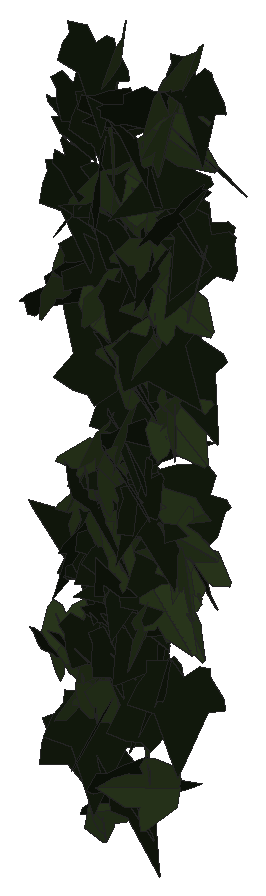
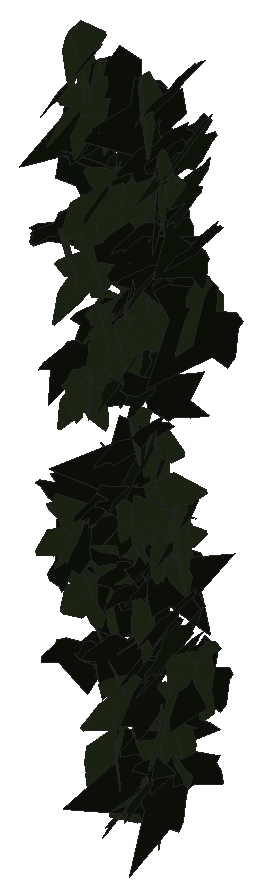
# SketchUp Ruby script. Lengths in inches.
U = 1.inch
M = Sketchup.active_model
def pt(a) = Geom::Point3d.new(a.map { |v| v * U })
def face(e, loops, mat)
  f = e.add_face(loops[0].map { |a| pt(a) })
  loops[1..].each { |l| e.add_face(l.map { |a| pt(a) }).erase! }
  f.material = f.back_material = mat if mat
  f
end
# faces: each face lists its corners as indices into pts; further lists are holes
def faces(e, pts, list, mat = nil) = list.each { |f| face(e, (f[0].is_a?(Array) ? f : [f]).map { |l| l.map { |i| pts[i] } }, mat) }
# xy, xz, yz: faces in a plane at the given z, y or x. An outline is a flat list of corners, or four numbers for a rectangle; further outlines are holes
def ring(l) = l.size == 4 ? [[l[0], l[1]], [l[2], l[1]], [l[2], l[3]], [l[0], l[3]]] : l.each_slice(2).to_a
def flat(e, list, mat, &to3) = list.each { |f| face(e, (f[0].is_a?(Array) ? f : [f]).map { |l| ring(l).map { |u, v| to3.(u, v) } }, mat) }
def xy(e, z, list, mat = nil) = flat(e, list, mat) { |x, y| [x, y, z] }
def xz(e, y, list, mat = nil) = flat(e, list, mat) { |x, z| [x, y, z] }
def yz(e, x, list, mat = nil) = flat(e, list, mat) { |y, z| [x, y, z] }
def lines(e, pts, list) = list.each { |a, b| e.add_line(pt(pts[a]), pt(pts[b])) }
# prism: a flat outline (further loops are holes) pulled along v
def prism(e, loops, v, mat = nil)
  f = face(e, loops, mat); d = Geom::Vector3d.new(v.map { |x| x * U })
  f.pushpull(f.normal.samedirection?(d) ? d.length : -d.length)
end
def box(e, o, s, mat = nil) = prism(e, [[o, [o[0] + s[0], o[1], o[2]], [o[0] + s[0], o[1] + s[1], o[2]], [o[0], o[1] + s[1], o[2]]]], [0, 0, s[2]], mat)
def at(x, y, z, deg = 0) = Geom::Transformation.translation(pt([x, y, z])) * Geom::Transformation.rotation(ORIGIN, Z_AXIS, deg.degrees)
def axes(o, x, y, z) = Geom::Transformation.new([*x, 0, *y, 0, *z, 0, *pt(o).to_a, 1])
def part(name) = M.definitions.add(name)
# library, detail: a bought-in or finely detailed component or shape, given as its bounding box
def library(name, o, s) = part(name).tap { |d| box(d.entities, o, s) }
def detail(e, o, s) = box(e.add_group.entities, o, s)
def put(e, d, t, mat = nil) = e.add_instance(d, t).tap { |i| i.material = mat if mat }
def group(e, t, mat = nil) = e.add_group.tap { |g| g.transformation = t; g.material = mat if mat }.entities
root = M.entities
M.materials.add("efeu1").color = [18, 25, 13]
M.materials.add("efeu2").color = [43, 57, 29]
c1 = part("ivyleaf_10")
p = [[0,0.5,-0.03],[-0.0625,2.02,-0.43],[-0.19,2.01,-0.46],[-0.54,1.05,-0.29],[-0.52,0.625,-0.18],[-0.83,0.76,-0.28],
  [-1.16,0.64,-0.33],[-1.15,0.33,-0.24],[-0.77,-0.39,0.02],[-0.3,-0.51,0.16],[0.04,-0.48,0.23],[-0.02,2.01,-0.4375],
  [-0.06,2.01,-0.43],[0.04,-0.49,0.23],[0.67,-0.49,0.14],[1.38,0.36,-0.2],[1.375,0.51,-0.24],[0.81,0.65,-0.19],
  [0.62,0.59,-0.15],[0.6,1.09,-0.28],[0.5,1.23,-0.31]]
faces(c1.entities,p,[[0,1,2,3,4,5,6,7,8,9,10],[11,12,0,13,14,15,16,17,18,19,20]],"efeu2")
c2 = part("ivyleaf_9")
p = [[1.54,2.16,1.25],[1.36,2.04,1.19],[-0.21,0.99,0.68],[-0.71,1.11,0.82],[-0.85,0.86,0.67],[-0.8,0.17,0.21],
  [-0.9,-0.01,0.1],[-0.67,-0.16,-0.02],[-0.08,-0.08,-0.05],[-0.03,-0.6,-0.4],[0.65,-0.88,-0.66],[0.83,-0.6,-0.49],
  [1.29,-0.42,-0.43],[1.8125,-0.07,-0.26],[1.21,0.44,0.15]]
faces(c2.entities,p,[[0,1,2,3,4,5,6,7,8,9,10,11,12,13,14]],"efeu1")
put(root,c1,axes([531.04,134.63,192.66],[0.26361,-0.71139,-0.19754],[-0.06426,0.18685,-0.75865],[0.73551,0.27129,0.00452]))
put(root,c2,axes([530.74,133.59,188.14],[0.75303,0.05984,-0.12105],[-0.12035,-0.01367,-0.75539],[-0.06125,0.76257,-0.00404]))
put(root,c2,axes([530.68,134.68,201.09],[0.16312,-0.82332,-0.03787],[-0.0011,0.03838,-0.8393],[0.82419,0.16299,0.00638]))
put(root,c2,axes([530.67,135.42,189.45],[0.04193,-0.62521,0.47513],[0.1896,-0.45367,-0.6137],[0.76203,0.14728,0.12655]))
put(root,c2,axes([530.9,133.39,198.6],[0.47981,0.7112,0.3862],[0.22324,0.31524,-0.85788],[-0.77789,0.52914,-0.00799]))
put(root,c1,axes([531.09,133.39,198.99],[-0.052,-0.49853,-0.72888],[0.08284,0.72417,-0.50121],[0.87917,-0.09772,0.00412]))
put(root,c1,axes([530.52,134.08,187.91],[0.10779,-0.17311,0.79881],[0.78917,-0.1877,-0.14717],[0.21277,0.78389,0.14117]))
put(root,c2,axes([531.32,133.77,200.6875],[0.21484,0.45839,0.65824],[0.01162,0.67959,-0.47705],[-0.80204,0.13264,0.16941]))
put(root,c1,axes([531.1,133.67,188.23],[0.32155,0.28852,-0.63424],[0.19396,0.63384,0.38668],[0.66924,-0.32233,0.19267]))
put(root,c1,axes([531.3,134.66,192.12],[-0.11723,-0.743,0.24242],[0.02821,-0.249,-0.74951],[0.78104,-0.10253,0.06345]))
put(root,c2,axes([531.81,134.42,190.58],[-0.00979,0.0925,0.81453],[-0.81733,0.06158,-0.01681],[-0.06308,-0.81226,0.09148]))
put(root,c2,axes([530.92,134.39,203.95],[0.45755,-0.69505,-0.09896],[-0.04108,0.09141,-0.83198],[0.70085,0.45912,0.01584]))
put(root,c2,axes([531.51,134.39,191.29],[-0.22531,0.51676,-0.53556],[0.20531,-0.49469,-0.5637],[-0.71534,-0.30475,0.00689]))
put(root,c1,axes([531.23,135.18,186.88],[-0.20489,0.5131,-0.49031],[0.08671,-0.48841,-0.54735],[-0.70438,-0.20937,0.07524]))
put(root,c2,axes([531.09,134.95,190.23],[0.19405,-0.73731,-0.05239],[-0.01151,0.05115,-0.76241],[0.73908,0.19438,0.00188]))
put(root,c1,axes([531.49,134.24,186.61],[0.08974,-0.89177,0.10539],[0.0243,-0.10347,-0.89616],[0.89764,0.09195,0.01373]))
put(root,c1,axes([531.67,134.61,193.43],[-0.44438,-0.65768,0.26278],[-0.05845,-0.27511,-0.78738],[0.70582,-0.43686,0.10025]))
put(root,c2,axes([532.08,134.54,196.17],[-0.78986,-0.33319,-0.19865],[-0.16849,-0.11122,0.8565],[-0.34941,0.80683,0.03603]))
put(root,c1,axes([531.67,134.48,191.43],[-0.44472,0.70787,-0.06223],[-0.0388,0.04911,0.83595],[0.70954,0.44635,0.00671]))
put(root,c2,axes([531.26,134.28,185.53],[-0.20793,-0.59761,-0.51311],[0.2079,0.47022,-0.63191],[0.75973,-0.29224,0.03249]))
put(root,c2,axes([531.3,133.41,203.66],[0.75435,-0.07109,-0.35592],[-0.28107,0.40497,-0.6766],[0.22964,0.7292,0.34106]))
put(root,c2,axes([531.41,134.5,184.7],[0.76234,-0.0328,-0.37748],[-0.37478,0.05955,-0.76205],[0.05577,0.84859,0.03888]))
put(root,c2,axes([531.26,133.6875,202.3],[0.65749,-0.42141,-0.2776],[-0.15246,0.26875,-0.76907],[0.48104,0.66116,0.13568]))
put(root,c1,axes([531.87,133.5625,187.26],[-0.12224,0.26561,0.72242],[-0.37787,0.61655,-0.29062],[-0.67056,-0.39585,0.03207]))
put(root,c2,axes([531.15,134.58,192.52],[0.54429,-0.78141,0.18703],[0.09921,-0.15881,-0.95225],[0.79733,0.55318,-0.00919]))
put(root,c2,axes([531.48,134.15,188.61],[0.36869,-0.62159,-0.33271],[-0.06126,0.34579,-0.71392],[0.70237,0.35645,0.11238]))
put(root,c2,axes([532.01,133.43,185.53],[0.05249,0.44209,0.63564],[0.02991,0.63547,-0.44444],[-0.77368,0.05456,0.02594]))
put(root,c2,axes([531.58,134.4,205.38],[0.10788,-0.82442,0.12259],[0.03031,-0.11965,-0.83133],[0.83294,0.11113,0.01438]))
put(root,c2,axes([531.61,134.8,191.22],[0.18444,-0.76454,-0.04074],[-0.00089,0.04169,-0.78642],[0.76562,0.18423,0.0089]))
put(root,c1,axes([532.01,134.82,205.35],[0.31164,-0.76022,-0.18841],[-0.00721,0.19998,-0.81884],[0.78318,0.30434,0.06744]))
put(root,c1,axes([532.11,134.15,202.97],[0.62794,-0.42437,-0.34252],[-0.13933,0.38019,-0.72647],[0.52725,0.60587,0.21595]))
put(root,c1,axes([532.32,133.64,183.4],[-0.12445,0.42105,-0.59435],[-0.26445,0.5357,0.43488],[0.67868,0.28594,0.06046]))
put(root,c2,axes([532.43,133.46,202.3],[0.03549,0.0188,-0.84588],[-0.74612,0.39992,-0.02242],[0.39897,0.74622,0.03332]))
put(root,c2,axes([531.92,134.18,186.125],[-0.28677,-0.81797,-0.1913],[0.07166,0.17758,-0.86674],[0.83698,-0.29546,0.00866]))
put(root,c1,axes([532.15,134.09,194.47],[0.06954,-0.75524,-0.18981],[0.03256,0.19322,-0.75687],[0.77804,0.05942,0.04864]))
put(root,c2,axes([531.78,134.27,199.75],[-0.04392,-0.58968,-0.56458],[0.19988,0.54042,-0.58],[0.79153,-0.16919,0.11513]))
put(root,c2,axes([532.61,135.1875,200.28],[-0.2321,-0.07874,0.763],[-0.71754,-0.25948,-0.24505],[0.27112,-0.75413,0.00465]))
put(root,c2,axes([531.8,134.7,201.48],[0.13318,-0.79396,-0.27331],[0.02514,0.28038,-0.80223],[0.83931,0.11759,0.0674]))
put(root,c2,axes([531.91,134.52,203.66],[0.02856,-0.81659,-0.19197],[-0.02894,0.19101,-0.81681],[0.83835,0.03441,-0.02166]))
put(root,c1,axes([531.91,134.41,191.91],[-0.50659,0.31057,-0.50559],[0.35044,-0.37986,-0.58447],[-0.47882,-0.6066,0.10715]))
put(root,c1,axes([532,134.92,189.29],[0.06572,-0.35407,-0.79019],[0.12113,-0.78091,0.35999],[-0.85738,-0.13747,-0.00971]))
put(root,c1,axes([532.29,134.93,193.07],[0.02918,-0.79936,0.0857],[0.00696,-0.0855,-0.79989],[0.80391,0.02976,0.00381]))
put(root,c2,axes([531.875,134.6875,199.97],[0.52852,-0.60117,-0.18155],[-0.0864,0.16542,-0.7993],[0.62202,0.53379,0.04324]))
put(root,c1,axes([532.4,134.27,186.95],[-0.49121,-0.65682,0.02553],[-0.01525,-0.02047,-0.82018],[0.65714,-0.49144,0.00004]))
put(root,c2,axes([532.77,135.22,193.18],[-0.61578,-0.06983,0.43979],[-0.42106,-0.15294,-0.61384],[0.14492,-0.74109,0.08524]))
put(root,c1,axes([532.6,134.06,191.27],[0.53556,-0.23189,-0.50994],[-0.47349,0.18962,-0.58351],[0.29936,0.71478,-0.01063]))
put(root,c1,axes([532.1875,134.09,198.66],[-0.26712,-0.54805,-0.55714],[0.29128,0.47655,-0.60842],[0.72521,-0.39327,0.03916]))
put(root,c1,axes([532.48,134.04,202],[-0.30002,-0.84663,0.00578],[-0.00184,-0.00548,-0.89821],[0.84665,-0.30002,0.0001]))
put(root,c2,axes([532.01,134.56,184.82],[0.51688,-0.65093,-0.05961],[-0.03879,0.04531,-0.83118],[0.6525,0.51833,-0.0022]))
put(root,c2,axes([531.99,135.25,194.22],[0.27883,-0.66473,0.43253],[0.147,-0.40722,-0.7206],[0.77932,0.31464,-0.01883]))
put(root,c1,axes([532.08,134.1,197.89],[0.68651,0.11248,-0.49154],[0.48576,0.07522,0.69565],[0.13527,-0.84098,-0.00352]))
put(root,c2,axes([531.96,134.53,187.5625],[0.82858,-0.34182,0.18948],[0.16868,-0.08788,-0.89616],[0.35254,0.84541,-0.01654]))
put(root,c2,axes([532.42,134.72,190.6],[-0.16663,-0.761,0.11539],[-0.00295,-0.11743,-0.77872],[0.76969,-0.1652,0.02199]))
put(root,c2,axes([532.19,134.58,200.71],[0.21458,-0.77793,0.15754],[0.07278,-0.14323,-0.80637],[0.79038,0.22439,0.03148]))
put(root,c2,axes([532.35,134.95,195.01],[-0.03554,-0.79116,-0.10623],[0.01827,0.1055,-0.79184],[0.79805,-0.03765,0.0134]))
put(root,c2,axes([532.39,134.5,190.86],[-0.31651,-0.60485,-0.43687],[0.18613,0.39554,-0.68248],[0.72253,-0.36686,-0.01556]))
put(root,c2,axes([532.23,134.58,193.125],[0.43206,-0.62245,-0.24071],[-0.07004,0.24287,-0.75377],[0.66368,0.43085,0.07715]))
put(root,c1,axes([532.7,133.45,193.68],[-0.18292,0.53797,0.53709],[-0.22845,0.48799,-0.56659],[-0.72505,-0.28948,0.04302]))
put(root,c2,axes([532.34,134.22,188.34],[0.30193,-0.69926,-0.17699],[-0.08116,0.15771,-0.76157],[0.71672,0.31243,-0.01169]))
put(root,c2,axes([532.14,134.38,196.73],[0.59211,-0.54134,0.14898],[0.11064,-0.09978,-0.80227],[0.55046,0.60235,0.001]))
put(root,c2,axes([532.73,134.27,189.03],[0.62248,-0.05553,0.53195],[-0.52657,0.07936,0.62447],[-0.09369,-0.81496,0.02456]))
put(root,c2,axes([532.11,133.76,203.85],[0.55006,0.15062,0.6169],[0.57939,0.21502,-0.56911],[-0.25992,0.79806,0.0369]))
put(root,c1,axes([532.38,133.58,183.77],[-0.0735,-0.08981,-0.73061],[0.46458,0.56387,-0.11605],[0.57098,-0.47036,0.00038]))
put(root,c1,axes([532.86,134.39,201.42],[-0.76252,-0.26645,0.11069],[-0.11263,-0.01306,-0.80736],[0.26564,-0.7704,-0.0246]))
put(root,c1,axes([532.68,134.33,194.93],[0.37753,-0.68155,0.1673],[0.08185,-0.14592,-0.77912],[0.69699,0.3863,0.00087]))
put(root,c2,axes([532.58,134.81,188.84],[-0.11024,-0.68489,-0.45434],[0.08855,0.44584,-0.69357],[0.8171,-0.14072,0.01386]))
put(root,c2,axes([532.36,134.39,193.38],[0.28643,-0.50862,0.53213],[0.30968,-0.43475,-0.58223],[0.6678,0.41976,0.04176]))
put(root,c1,axes([532.59,134.5,187.11],[-0.34134,-0.27715,-0.64569],[0.5212,0.38158,-0.43931],[0.47126,-0.62276,0.01818]))
put(root,c2,axes([532.4,134.35,193.83],[0.43906,0.11727,0.70979],[0.6632,0.25625,-0.45257],[-0.27878,0.7943,0.04121]))
put(root,c1,axes([533.08,134.81,197.66],[-0.34941,-0.67022,0.29406],[-0.00808,-0.3223,-0.74419],[0.73185,-0.32355,0.13218]))
put(root,c2,axes([532.56,133.5,184.28],[0.52369,0.38051,0.68488],[0.53127,0.43301,-0.6468],[-0.57585,0.74553,0.02611]))
put(root,c2,axes([532.51,134.52,203.12],[0.16561,-0.57207,0.58879],[0.30832,-0.51334,-0.58548],[0.76084,0.33254,0.1091]))
put(root,c2,axes([532.82,133.9375,199.03],[0.37706,-0.51834,-0.57077],[-0.29889,0.48742,-0.64009],[0.71072,0.47998,0.03362]))
put(root,c2,axes([532.625,134.56,184.05],[0.35268,-0.73903,0.03827],[0.01741,-0.0341,-0.81887],[0.73981,0.3531,0.00102]))
put(root,c2,axes([533.66,134.49,190.55],[-0.71863,0.06407,0.43761],[-0.4387,0.00266,-0.72081],[-0.05611,-0.84138,0.03104]))
put(root,c2,axes([532.9,134.83,188.45],[-0.29988,-0.57735,0.46408],[0.09329,-0.52612,-0.59425],[0.73485,-0.16882,0.26482]))
put(root,c2,axes([532.5625,134.54,192.59],[0.7129,-0.30211,0.154],[0.13724,-0.07078,-0.77419],[0.31008,0.7259,-0.01139]))
put(root,c1,axes([533.13,134.39,198.24],[-0.01812,-0.74129,0.37323],[0.07153,-0.37332,-0.738],[0.82685,0.01605,0.07202]))
put(root,c1,axes([533.38,133.91,197.1],[-0.73795,-0.28634,0.22004],[-0.18699,-0.12528,-0.79014],[0.30893,-0.7598,0.04736]))
put(root,c1,axes([532.74,134.98,185.38],[0.0457,-0.17408,0.78669],[0.64452,-0.46496,-0.14033],[0.48351,0.63623,0.1127]))
put(root,c2,axes([532.8,134.74,196.67],[0.3601,-0.7032,0.15678],[0.04934,-0.15079,-0.78967],[0.71878,0.36265,-0.02434]))
put(root,c1,axes([533.77,134.38,184.51],[-0.06632,-0.04578,-0.84309],[-0.68978,-0.48478,0.08058],[-0.48693,0.69296,0.00067]))
put(root,c1,axes([533.21,134.59,190.77],[-0.78939,-0.00174,0.28742],[0.28741,-0.01148,0.78931],[0.00229,0.84001,0.01138]))
put(root,c2,axes([532.97,134.47,199.91],[-0.18167,-0.01208,-0.80373],[0.80324,-0.03401,-0.18105],[-0.03052,-0.8233,0.01927]))
put(root,c1,axes([533.06,134.36,201.91],[0.31289,0.39375,0.66475],[0.31185,0.59181,-0.49733],[-0.70688,0.43537,0.07483]))
put(root,c1,axes([533.34,134.38,189.4],[0.22751,-0.53815,0.4661],[0.18161,-0.42926,-0.58427],[0.68838,0.29111,0.0001]))
put(root,c2,axes([532.9375,134.26,196.24],[0.15952,-0.47445,0.62182],[0.34231,-0.52827,-0.49088],[0.70327,0.36475,0.09789]))
put(root,c2,axes([533.27,133.53,204.66],[0.61215,0.56513,0.13133],[0.10192,0.08321,-0.83309],[-0.57117,0.62053,-0.0079]))
put(root,c2,axes([533.53,134.11,193.49],[-0.67997,0.05996,-0.41279],[0.4092,-0.05723,-0.68237],[-0.0809,-0.7934,0.01802]))
put(root,c1,axes([533.59,134.88,201.39],[-0.4892,-0.66717,0.05283],[0.00877,-0.07182,-0.82582],[0.6692,-0.48678,0.04944]))
put(root,c2,axes([534.14,133.9,187.18],[-0.71524,-0.34201,-0.38711],[-0.35103,-0.16323,0.7928],[-0.37895,0.79673,-0.00375]))
put(root,c2,axes([533.21,134.42,192.91],[0.21375,-0.72505,-0.31162],[-0.04802,0.3103,-0.75492],[0.78772,0.21566,0.03854]))
put(root,c1,axes([533.58,135.27,204.37],[0.04112,0.43246,-0.78849],[-0.12417,-0.77903,-0.43374],[-0.89069,0.12857,0.02407]))
put(root,c1,axes([533.71,134.02,200.38],[-0.6578,-0.4557,-0.05778],[0.05922,0.01594,-0.79996],[0.45551,-0.66014,0.02057]))
put(root,c2,axes([534.0625,133.75,200.0625],[-0.57294,0.562,-0.04025],[0.02798,-0.02896,-0.80256],[-0.56274,-0.57362,0.00108]))
put(root,c2,axes([533.45,134.43,192.8],[0.08878,-0.78102,-0.2264],[0.00177,0.22793,-0.7856],[0.81317,0.08478,0.02643]))
put(root,c2,axes([533.77,134.28,188.06],[-0.59956,0.14142,-0.49329],[0.47155,-0.14744,-0.6154],[-0.20244,-0.76228,0.02751]))
put(root,c2,axes([533.38,134.7,202.13],[0.56744,-0.60299,-0.06393],[-0.04009,0.05006,-0.82798],[0.60504,0.56883,0.0051]))
put(root,c1,axes([533.5,133.77,197.72],[-0.36374,-0.44049,-0.55113],[0.53527,0.23167,-0.53843],[0.45964,-0.61838,0.19087]))
put(root,c1,axes([533.9375,133.82,197.85],[-0.06924,-0.61189,-0.50447],[0.06578,0.50021,-0.61575],[0.79029,-0.09524,0.00705]))
put(root,c1,axes([533.92,134.24,204.93],[0.1839,-0.76296,-0.31972],[0.06753,0.34027,-0.77318],[0.82448,0.14231,0.13464]))
put(root,c1,axes([534.46,134.71,192.52],[-0.29732,-0.25344,0.69395],[-0.55969,-0.411,-0.3899],[0.48223,-0.63328,-0.02467]))
put(root,c2,axes([534.41,134.72,202.57],[-0.82319,-0.03754,0.13475],[-0.11895,-0.23536,-0.79225],[0.0736,-0.80025,0.22668]))
put(root,c2,axes([533.77,133.82,197.84],[0.05753,-0.47721,-0.63361],[0.05721,0.63611,-0.4739],[0.79115,-0.0113,0.08034]))
put(root,c2,axes([534.57,135.14,192.99],[-0.75264,-0.21323,0.16253],[-0.15397,-0.05276,-0.78221],[0.21949,-0.76818,0.00861]))
put(root,c1,axes([534.31,133.93,204.27],[0.1836,-0.81684,-0.06645],[-0.01169,0.06548,-0.83722],[0.81945,0.18395,0.00295]))
put(root,c1,axes([533.92,134.2,190.08],[-0.55913,-0.23857,-0.44204],[0.49765,-0.17329,-0.53596],[0.0682,-0.69137,0.28686]))
put(root,c1,axes([534.35,134.5,195.84],[0.0627,-0.74217,0.31287],[0.00039,-0.31379,-0.74442],[0.80542,0.05793,-0.024]))
put(root,c1,axes([534.22,134.125,199.11],[0.10667,0.64739,0.59586],[0.06357,0.59298,-0.65564],[-0.87756,0.12165,0.02493]))
put(root,c1,axes([533.78,134.53,192.04],[-0.18621,0.06267,-0.81817],[0.79411,-0.19756,-0.19586],[-0.20669,-0.81551,-0.01542]))
put(root,c1,axes([534.46,134.59,205.79],[0.15308,-0.82908,0.14199],[0.01115,-0.14231,-0.84297],[0.84108,0.15278,-0.01467]))
put(root,c2,axes([534.12,134.75,197.0625],[0.08847,-0.69389,-0.44416],[-0.00849,0.44592,-0.69833],[0.82383,0.07911,0.0405]))
put(root,c1,axes([534.05,134.42,195.93],[0.14503,-0.50452,0.59318],[0.53452,-0.37428,-0.44903],[0.56629,0.4825,0.27193]))
put(root,c1,axes([533.91,134.83,189.72],[0.47765,-0.02765,0.635],[0.6331,-0.0497,-0.47838],[0.05633,0.79303,-0.00784]))
put(root,c1,axes([534.2,133.96,203.92],[-0.54789,-0.30516,-0.59299],[0.49849,0.32242,-0.6265],[0.44302,-0.74018,-0.02842]))
put(root,c1,axes([534.41,134.58,191.27],[-0.14883,0.72588,-0.13156],[0.02519,-0.12913,-0.74098],[-0.73728,-0.15095,0.00124]))
put(root,c1,axes([534.53,134.73,191.27],[0.60057,0.41047,-0.19109],[-0.1919,-0.05674,-0.72501],[-0.41009,0.62768,0.05942]))
put(root,c2,axes([534.8,133.53,202.03],[-0.12495,0.81723,-0.06658],[0.01699,-0.06475,-0.8267],[-0.81976,-0.12591,-0.00699]))
put(root,c2,axes([534.08,134.61,203.75],[0.77511,-0.32673,-0.013],[0.03274,0.11084,-0.83328],[0.32534,0.76726,0.11484]))
put(root,c1,axes([534.32,133.99,195.62],[0.28338,0.58866,0.45523],[0.20148,0.40824,-0.65331],[-0.71636,0.34768,-0.00366]))
put(root,c2,axes([534.5625,135.27,200.83],[-0.3342,-0.69655,0.2395],[-0.03706,-0.24677,-0.76939],[0.73564,-0.32887,0.07005]))
put(root,c2,axes([534.28,135.08,205.0625],[0.18092,-0.79373,0.16353],[0.00787,-0.16583,-0.81359],[0.81037,0.17882,-0.02861]))
put(root,c2,axes([534.48,134.3,187.91],[-0.35768,-0.70087,-0.2783],[0.11835,0.25203,-0.78682],[0.74476,-0.37666,-0.00862]))
put(root,c2,axes([534.18,135.15,190.69],[-0.02344,-0.27847,0.74599],[0.35241,-0.67287,-0.2401],[0.71404,0.32294,0.14299]))
put(root,c2,axes([534.74,135.01,200.65],[-0.45203,-0.66334,0.09907],[-0.05547,-0.08209,-0.80272],[0.6684,-0.45542,0.00039]))
put(root,c1,axes([534.62,134.83,200.01],[0.54459,-0.59183,0.15873],[0.11958,-0.10563,-0.8041],[0.60097,0.55733,0.01615]))
